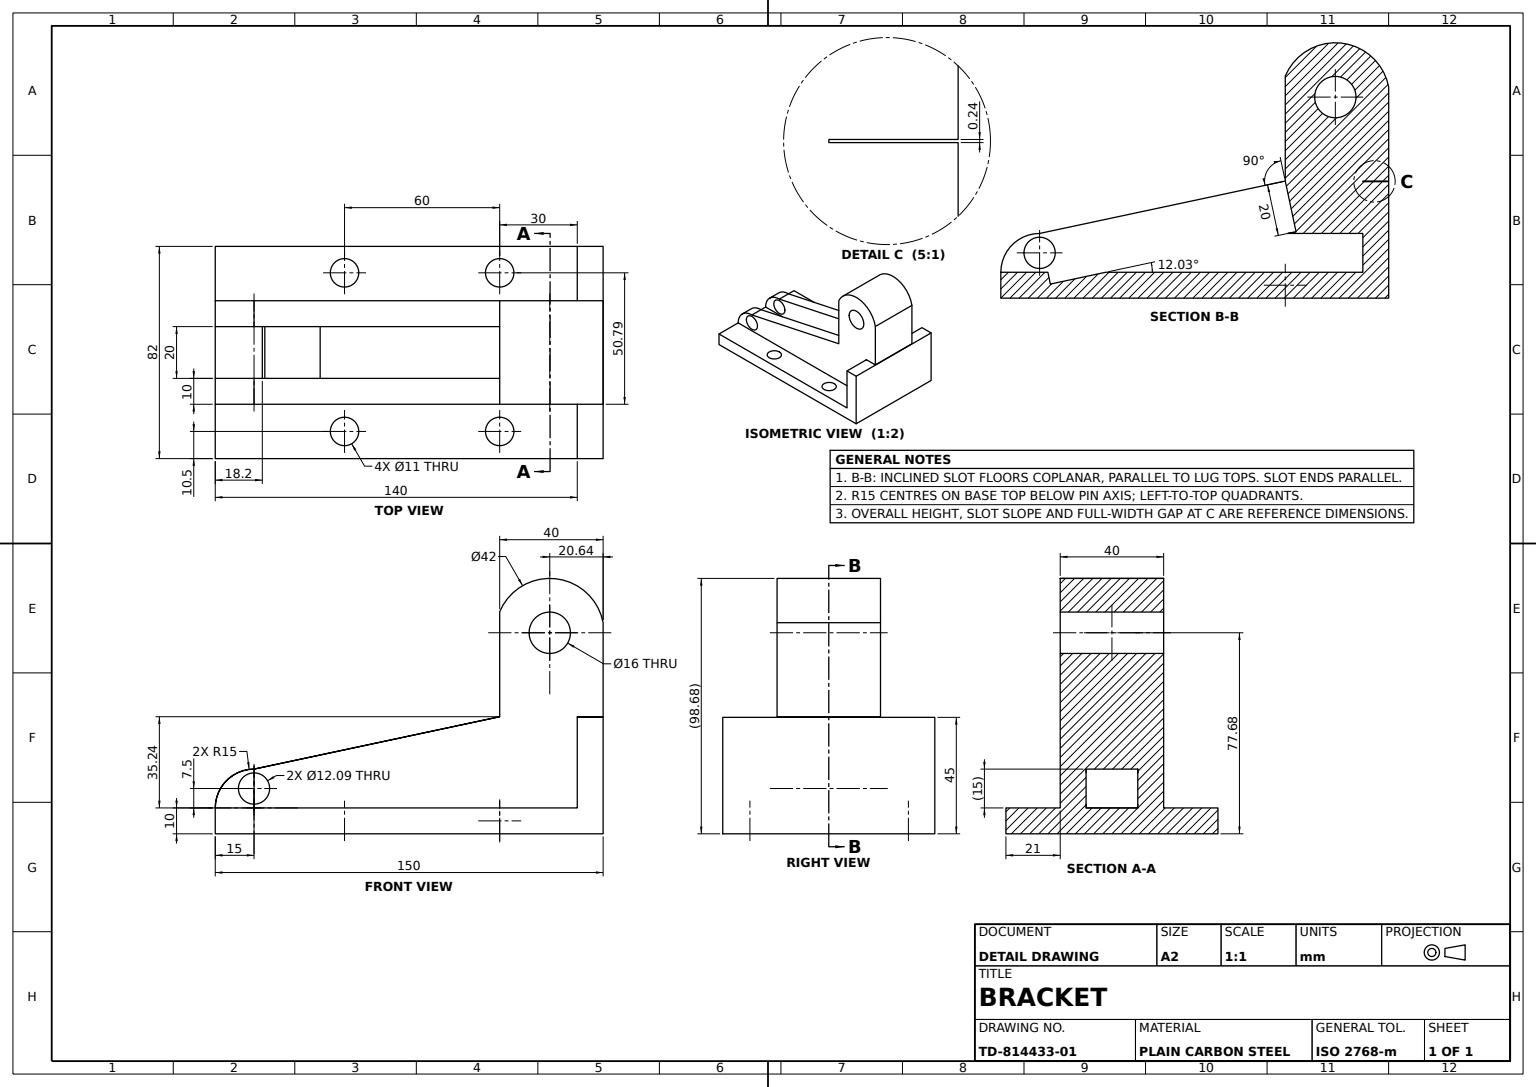
ISO-10303-21;
HEADER;
FILE_DESCRIPTION((''),'2;1');
FILE_NAME('','',(''),(''),'','','');
FILE_SCHEMA(('AUTOMOTIVE_DESIGN'));
ENDSEC;
DATA;
#1=APPLICATION_CONTEXT('');
#2=PRODUCT_CONTEXT('',#1,'mechanical');
#3=PRODUCT('','','',(#2));
#4=PRODUCT_DEFINITION_FORMATION('','',#3);
#5=PRODUCT_DEFINITION_CONTEXT('',#1,'design');
#6=PRODUCT_DEFINITION('','',#4,#5);
#7=PRODUCT_DEFINITION_SHAPE('','',#6);
#8=(LENGTH_UNIT()NAMED_UNIT(*)SI_UNIT(.MILLI.,.METRE.));
#9=(NAMED_UNIT(*)PLANE_ANGLE_UNIT()SI_UNIT($,.RADIAN.));
#10=(NAMED_UNIT(*)SI_UNIT($,.STERADIAN.)SOLID_ANGLE_UNIT());
#11=UNCERTAINTY_MEASURE_WITH_UNIT(LENGTH_MEASURE(1.E-05),#8,'distance_accuracy_value','');
#12=(GEOMETRIC_REPRESENTATION_CONTEXT(3)GLOBAL_UNCERTAINTY_ASSIGNED_CONTEXT((#11))GLOBAL_UNIT_ASSIGNED_CONTEXT((#8,#9,#10))REPRESENTATION_CONTEXT('',''));
#13=CARTESIAN_POINT('',(18.196186,10.,10.));
#14=VERTEX_POINT('',#13);
#15=CARTESIAN_POINT('',(0.,10.,10.));
#16=VERTEX_POINT('',#15);
#17=DIRECTION('',(-1.,0.,0.));
#18=VECTOR('',#17,1000.);
#19=LINE('',#15,#18);
#20=EDGE_CURVE('',#14,#16,#19,.T.);
#21=ORIENTED_EDGE('',*,*,#20,.F.);
#22=CARTESIAN_POINT('',(18.196186,10.,-10.));
#23=VERTEX_POINT('',#22);
#24=CARTESIAN_POINT('',(18.196186,10.,41.));
#25=DIRECTION('',(0.,0.,-1.));
#26=VECTOR('',#25,1000.);
#27=LINE('',#24,#26);
#28=EDGE_CURVE('',#14,#23,#27,.T.);
#29=ORIENTED_EDGE('',*,*,#28,.T.);
#30=CARTESIAN_POINT('',(0.,10.,-10.));
#31=VERTEX_POINT('',#30);
#32=DIRECTION('',(1.,0.,0.));
#33=VECTOR('',#32,1000.);
#34=LINE('',#30,#33);
#35=EDGE_CURVE('',#31,#23,#34,.T.);
#36=ORIENTED_EDGE('',*,*,#35,.F.);
#37=CARTESIAN_POINT('',(0.,10.,41.));
#38=LINE('',#37,#26);
#39=EDGE_CURVE('',#16,#31,#38,.T.);
#40=ORIENTED_EDGE('',*,*,#39,.F.);
#41=EDGE_LOOP('',(#21,#29,#36,#40));
#42=FACE_OUTER_BOUND('',#41,.T.);
#43=DIRECTION('',(0.,-1.,0.));
#44=AXIS2_PLACEMENT_3D('',#37,#43,#25);
#45=PLANE('',#44);
#46=ADVANCED_FACE('',(#42),#45,.F.);
#47=CARTESIAN_POINT('',(110.,45.24251,-10.));
#48=VERTEX_POINT('',#47);
#49=CARTESIAN_POINT('',(15.,25.,-10.));
#50=VERTEX_POINT('',#49);
#51=DIRECTION('',(-0.978043553,-0.208400594,0.));
#52=VECTOR('',#51,1000.);
#53=LINE('',#49,#52);
#54=EDGE_CURVE('',#48,#50,#53,.T.);
#55=ORIENTED_EDGE('',*,*,#54,.F.);
#56=CARTESIAN_POINT('',(110.,45.24251,-20.));
#57=VERTEX_POINT('',#56);
#58=LINE('',#47,#26);
#59=EDGE_CURVE('',#48,#57,#58,.T.);
#60=ORIENTED_EDGE('',*,*,#59,.T.);
#61=CARTESIAN_POINT('',(15.,25.,-20.));
#62=VERTEX_POINT('',#61);
#63=DIRECTION('',(0.978043553,0.208400594,0.));
#64=VECTOR('',#63,1000.);
#65=LINE('',#56,#64);
#66=EDGE_CURVE('',#62,#57,#65,.T.);
#67=ORIENTED_EDGE('',*,*,#66,.F.);
#68=DIRECTION('',(0.,0.,1.));
#69=VECTOR('',#68,1000.);
#70=LINE('',#49,#69);
#71=EDGE_CURVE('',#62,#50,#70,.T.);
#72=ORIENTED_EDGE('',*,*,#71,.T.);
#73=EDGE_LOOP('',(#55,#60,#67,#72));
#74=FACE_OUTER_BOUND('',#73,.T.);
#75=DIRECTION('',(-0.208400594,0.978043553,0.));
#76=AXIS2_PLACEMENT_3D('',#47,#75,#51);
#77=PLANE('',#76);
#78=ADVANCED_FACE('',(#74),#77,.T.);
#79=CARTESIAN_POINT('',(150.,45.,41.));
#80=VERTEX_POINT('',#79);
#81=CARTESIAN_POINT('',(140.,45.,41.));
#82=VERTEX_POINT('',#81);
#83=LINE('',#79,#18);
#84=EDGE_CURVE('',#80,#82,#83,.T.);
#85=ORIENTED_EDGE('',*,*,#84,.T.);
#86=CARTESIAN_POINT('',(140.,10.,41.));
#87=VERTEX_POINT('',#86);
#88=VECTOR('',#43,1000.);
#89=LINE('',#81,#88);
#90=EDGE_CURVE('',#82,#87,#89,.T.);
#91=ORIENTED_EDGE('',*,*,#90,.T.);
#92=VERTEX_POINT('',#37);
#93=LINE('',#37,#18);
#94=EDGE_CURVE('',#87,#92,#93,.T.);
#95=ORIENTED_EDGE('',*,*,#94,.T.);
#96=CARTESIAN_POINT('',(0.,0.,41.));
#97=VERTEX_POINT('',#96);
#98=LINE('',#96,#88);
#99=EDGE_CURVE('',#92,#97,#98,.T.);
#100=ORIENTED_EDGE('',*,*,#99,.T.);
#101=CARTESIAN_POINT('',(150.,0.,41.));
#102=VERTEX_POINT('',#101);
#103=LINE('',#96,#33);
#104=EDGE_CURVE('',#97,#102,#103,.T.);
#105=ORIENTED_EDGE('',*,*,#104,.T.);
#106=DIRECTION('',(0.,1.,0.));
#107=VECTOR('',#106,1000.);
#108=LINE('',#101,#107);
#109=EDGE_CURVE('',#102,#80,#108,.T.);
#110=ORIENTED_EDGE('',*,*,#109,.T.);
#111=EDGE_LOOP('',(#85,#91,#95,#100,#105,#110));
#112=FACE_OUTER_BOUND('',#111,.T.);
#113=AXIS2_PLACEMENT_3D('',#96,#25,#17);
#114=PLANE('',#113);
#115=ADVANCED_FACE('',(#112),#114,.F.);
#116=CARTESIAN_POINT('',(110.,85.812237,-20.));
#117=VERTEX_POINT('',#116);
#118=LINE('',#56,#107);
#119=EDGE_CURVE('',#57,#117,#118,.T.);
#120=ORIENTED_EDGE('',*,*,#119,.F.);
#121=ORIENTED_EDGE('',*,*,#59,.F.);
#122=CARTESIAN_POINT('',(110.,45.24251,10.));
#123=VERTEX_POINT('',#122);
#124=EDGE_CURVE('',#123,#48,#58,.T.);
#125=ORIENTED_EDGE('',*,*,#124,.F.);
#126=CARTESIAN_POINT('',(110.,45.24251,20.));
#127=VERTEX_POINT('',#126);
#128=EDGE_CURVE('',#127,#123,#58,.T.);
#129=ORIENTED_EDGE('',*,*,#128,.F.);
#130=CARTESIAN_POINT('',(110.,85.812237,20.));
#131=VERTEX_POINT('',#130);
#132=LINE('',#126,#107);
#133=EDGE_CURVE('',#127,#131,#132,.T.);
#134=ORIENTED_EDGE('',*,*,#133,.T.);
#135=LINE('',#116,#69);
#136=EDGE_CURVE('',#117,#131,#135,.T.);
#137=ORIENTED_EDGE('',*,*,#136,.F.);
#138=EDGE_LOOP('',(#120,#121,#125,#129,#134,#137));
#139=FACE_OUTER_BOUND('',#138,.T.);
#140=AXIS2_PLACEMENT_3D('',#56,#32,#25);
#141=PLANE('',#140);
#142=ADVANCED_FACE('',(#139),#141,.F.);
#143=CARTESIAN_POINT('',(0.,10.,-20.));
#144=VERTEX_POINT('',#143);
#145=CARTESIAN_POINT('',(0.,10.,-41.));
#146=VERTEX_POINT('',#145);
#147=EDGE_CURVE('',#144,#146,#38,.T.);
#148=ORIENTED_EDGE('',*,*,#147,.F.);
#149=CARTESIAN_POINT('',(140.,10.,-20.));
#150=VERTEX_POINT('',#149);
#151=LINE('',#143,#18);
#152=EDGE_CURVE('',#150,#144,#151,.T.);
#153=ORIENTED_EDGE('',*,*,#152,.F.);
#154=CARTESIAN_POINT('',(140.,10.,-41.));
#155=VERTEX_POINT('',#154);
#156=LINE('',#86,#26);
#157=EDGE_CURVE('',#150,#155,#156,.T.);
#158=ORIENTED_EDGE('',*,*,#157,.T.);
#159=LINE('',#145,#18);
#160=EDGE_CURVE('',#155,#146,#159,.T.);
#161=ORIENTED_EDGE('',*,*,#160,.T.);
#162=EDGE_LOOP('',(#148,#153,#158,#161));
#163=FACE_OUTER_BOUND('',#162,.T.);
#164=CARTESIAN_POINT('',(50.,10.,-25.288669));
#165=VERTEX_POINT('',#164);
#166=CARTESIAN_POINT('',(50.,10.,-36.28851));
#167=VERTEX_POINT('',#166);
#168=CARTESIAN_POINT('',(50.,10.,-30.788589));
#169=AXIS2_PLACEMENT_3D('',#168,#106,#68);
#170=CIRCLE('',#169,5.49992);
#171=EDGE_CURVE('',#165,#167,#170,.T.);
#172=ORIENTED_EDGE('',*,*,#171,.F.);
#173=EDGE_CURVE('',#167,#165,#170,.T.);
#174=ORIENTED_EDGE('',*,*,#173,.F.);
#175=EDGE_LOOP('',(#172,#174));
#176=FACE_BOUND('',#175,.T.);
#177=CARTESIAN_POINT('',(110.,10.,-25.288589));
#178=VERTEX_POINT('',#177);
#179=CARTESIAN_POINT('',(110.,10.,-36.288589));
#180=VERTEX_POINT('',#179);
#181=CARTESIAN_POINT('',(110.,10.,-30.788589));
#182=AXIS2_PLACEMENT_3D('',#181,#106,#68);
#183=CIRCLE('',#182,5.5);
#184=EDGE_CURVE('',#178,#180,#183,.T.);
#185=ORIENTED_EDGE('',*,*,#184,.F.);
#186=EDGE_CURVE('',#180,#178,#183,.T.);
#187=ORIENTED_EDGE('',*,*,#186,.F.);
#188=EDGE_LOOP('',(#185,#187));
#189=FACE_BOUND('',#188,.T.);
#190=ADVANCED_FACE('',(#163,#176,#189),#45,.F.);
#191=CARTESIAN_POINT('',(50.,0.,36.));
#192=VERTEX_POINT('',#191);
#193=CARTESIAN_POINT('',(50.,0.,25.));
#194=VERTEX_POINT('',#193);
#195=CARTESIAN_POINT('',(50.,0.,30.5));
#196=AXIS2_PLACEMENT_3D('',#195,#106,#68);
#197=CIRCLE('',#196,5.5);
#198=EDGE_CURVE('',#192,#194,#197,.T.);
#199=ORIENTED_EDGE('',*,*,#198,.T.);
#200=EDGE_CURVE('',#194,#192,#197,.T.);
#201=ORIENTED_EDGE('',*,*,#200,.T.);
#202=EDGE_LOOP('',(#199,#201));
#203=FACE_BOUND('',#202,.T.);
#204=CARTESIAN_POINT('',(110.,0.,-25.288589));
#205=VERTEX_POINT('',#204);
#206=CARTESIAN_POINT('',(110.,0.,-36.288589));
#207=VERTEX_POINT('',#206);
#208=CARTESIAN_POINT('',(110.,0.,-30.788589));
#209=AXIS2_PLACEMENT_3D('',#208,#106,#68);
#210=CIRCLE('',#209,5.5);
#211=EDGE_CURVE('',#205,#207,#210,.T.);
#212=ORIENTED_EDGE('',*,*,#211,.T.);
#213=EDGE_CURVE('',#207,#205,#210,.T.);
#214=ORIENTED_EDGE('',*,*,#213,.T.);
#215=EDGE_LOOP('',(#212,#214));
#216=FACE_BOUND('',#215,.T.);
#217=CARTESIAN_POINT('',(50.,0.,-25.288669));
#218=VERTEX_POINT('',#217);
#219=CARTESIAN_POINT('',(50.,0.,-36.28851));
#220=VERTEX_POINT('',#219);
#221=CARTESIAN_POINT('',(50.,0.,-30.788589));
#222=AXIS2_PLACEMENT_3D('',#221,#106,#68);
#223=CIRCLE('',#222,5.49992);
#224=EDGE_CURVE('',#218,#220,#223,.T.);
#225=ORIENTED_EDGE('',*,*,#224,.T.);
#226=EDGE_CURVE('',#220,#218,#223,.T.);
#227=ORIENTED_EDGE('',*,*,#226,.T.);
#228=EDGE_LOOP('',(#225,#227));
#229=FACE_BOUND('',#228,.T.);
#230=CARTESIAN_POINT('',(0.,0.,-41.));
#231=VERTEX_POINT('',#230);
#232=LINE('',#96,#26);
#233=EDGE_CURVE('',#97,#231,#232,.T.);
#234=ORIENTED_EDGE('',*,*,#233,.T.);
#235=CARTESIAN_POINT('',(150.,0.,-41.));
#236=VERTEX_POINT('',#235);
#237=LINE('',#230,#33);
#238=EDGE_CURVE('',#231,#236,#237,.T.);
#239=ORIENTED_EDGE('',*,*,#238,.T.);
#240=LINE('',#101,#26);
#241=EDGE_CURVE('',#102,#236,#240,.T.);
#242=ORIENTED_EDGE('',*,*,#241,.F.);
#243=ORIENTED_EDGE('',*,*,#104,.F.);
#244=EDGE_LOOP('',(#234,#239,#242,#243));
#245=FACE_OUTER_BOUND('',#244,.T.);
#246=CARTESIAN_POINT('',(110.,0.,36.));
#247=VERTEX_POINT('',#246);
#248=CARTESIAN_POINT('',(110.,0.,25.));
#249=VERTEX_POINT('',#248);
#250=CARTESIAN_POINT('',(110.,0.,30.5));
#251=AXIS2_PLACEMENT_3D('',#250,#106,#68);
#252=CIRCLE('',#251,5.5);
#253=EDGE_CURVE('',#247,#249,#252,.T.);
#254=ORIENTED_EDGE('',*,*,#253,.T.);
#255=EDGE_CURVE('',#249,#247,#252,.T.);
#256=ORIENTED_EDGE('',*,*,#255,.T.);
#257=EDGE_LOOP('',(#254,#256));
#258=FACE_BOUND('',#257,.T.);
#259=AXIS2_PLACEMENT_3D('',#96,#106,#68);
#260=PLANE('',#259);
#261=ADVANCED_FACE('',(#203,#216,#229,#245,#258),#260,.F.);
#262=CARTESIAN_POINT('',(50.,10.,25.));
#263=VERTEX_POINT('',#262);
#264=CARTESIAN_POINT('',(50.,-70.,25.));
#265=LINE('',#264,#107);
#266=EDGE_CURVE('',#194,#263,#265,.T.);
#267=ORIENTED_EDGE('',*,*,#266,.T.);
#268=CARTESIAN_POINT('',(50.,10.,36.));
#269=VERTEX_POINT('',#268);
#270=CARTESIAN_POINT('',(50.,10.,30.5));
#271=AXIS2_PLACEMENT_3D('',#270,#106,#68);
#272=CIRCLE('',#271,5.5);
#273=EDGE_CURVE('',#263,#269,#272,.T.);
#274=ORIENTED_EDGE('',*,*,#273,.T.);
#275=CARTESIAN_POINT('',(50.,-70.,36.));
#276=LINE('',#275,#107);
#277=EDGE_CURVE('',#192,#269,#276,.T.);
#278=ORIENTED_EDGE('',*,*,#277,.F.);
#279=ORIENTED_EDGE('',*,*,#200,.F.);
#280=EDGE_LOOP('',(#267,#274,#278,#279));
#281=FACE_OUTER_BOUND('',#280,.T.);
#282=CARTESIAN_POINT('',(50.,-70.,30.5));
#283=AXIS2_PLACEMENT_3D('',#282,#106,#68);
#284=CYLINDRICAL_SURFACE('',#283,5.5);
#285=ADVANCED_FACE('',(#281),#284,.F.);
#286=CARTESIAN_POINT('',(150.,45.24251,-20.));
#287=VERTEX_POINT('',#286);
#288=CARTESIAN_POINT('',(150.,45.24251,20.));
#289=VERTEX_POINT('',#288);
#290=LINE('',#286,#69);
#291=EDGE_CURVE('',#287,#289,#290,.T.);
#292=ORIENTED_EDGE('',*,*,#291,.F.);
#293=CARTESIAN_POINT('',(150.,81.572935,-20.));
#294=VERTEX_POINT('',#293);
#295=CARTESIAN_POINT('',(150.,90.24251,-20.));
#296=LINE('',#295,#88);
#297=EDGE_CURVE('',#294,#287,#296,.T.);
#298=ORIENTED_EDGE('',*,*,#297,.F.);
#299=CARTESIAN_POINT('',(150.,81.572935,20.));
#300=VERTEX_POINT('',#299);
#301=LINE('',#293,#69);
#302=EDGE_CURVE('',#294,#300,#301,.T.);
#303=ORIENTED_EDGE('',*,*,#302,.T.);
#304=CARTESIAN_POINT('',(150.,90.24251,20.));
#305=LINE('',#304,#88);
#306=EDGE_CURVE('',#300,#289,#305,.T.);
#307=ORIENTED_EDGE('',*,*,#306,.T.);
#308=EDGE_LOOP('',(#292,#298,#303,#307));
#309=FACE_OUTER_BOUND('',#308,.T.);
#310=AXIS2_PLACEMENT_3D('',#295,#17,#68);
#311=PLANE('',#310);
#312=ADVANCED_FACE('',(#309),#311,.F.);
#313=CARTESIAN_POINT('',(137.363208,77.684128,-20.));
#314=VERTEX_POINT('',#313);
#315=CARTESIAN_POINT('',(137.363208,77.684128,20.));
#316=VERTEX_POINT('',#315);
#317=LINE('',#313,#69);
#318=EDGE_CURVE('',#314,#316,#317,.T.);
#319=ORIENTED_EDGE('',*,*,#318,.F.);
#320=CARTESIAN_POINT('',(121.363208,77.684128,-20.));
#321=VERTEX_POINT('',#320);
#322=CARTESIAN_POINT('',(129.363208,77.684128,-20.));
#323=AXIS2_PLACEMENT_3D('',#322,#68,#32);
#324=CIRCLE('',#323,8.);
#325=EDGE_CURVE('',#321,#314,#324,.T.);
#326=ORIENTED_EDGE('',*,*,#325,.F.);
#327=CARTESIAN_POINT('',(121.363208,77.684128,20.));
#328=VERTEX_POINT('',#327);
#329=LINE('',#320,#69);
#330=EDGE_CURVE('',#321,#328,#329,.T.);
#331=ORIENTED_EDGE('',*,*,#330,.T.);
#332=CARTESIAN_POINT('',(129.363208,77.684128,20.));
#333=AXIS2_PLACEMENT_3D('',#332,#68,#32);
#334=CIRCLE('',#333,8.);
#335=EDGE_CURVE('',#328,#316,#334,.T.);
#336=ORIENTED_EDGE('',*,*,#335,.T.);
#337=EDGE_LOOP('',(#319,#326,#331,#336));
#338=FACE_OUTER_BOUND('',#337,.T.);
#339=CYLINDRICAL_SURFACE('',#323,8.);
#340=ADVANCED_FACE('',(#338),#339,.F.);
#341=ORIENTED_EDGE('',*,*,#152,.T.);
#342=CARTESIAN_POINT('',(15.,10.,-20.));
#343=AXIS2_PLACEMENT_3D('',#342,#25,#32);
#344=CIRCLE('',#343,15.);
#345=EDGE_CURVE('',#144,#62,#344,.T.);
#346=ORIENTED_EDGE('',*,*,#345,.T.);
#347=ORIENTED_EDGE('',*,*,#66,.T.);
#348=ORIENTED_EDGE('',*,*,#119,.T.);
#349=CIRCLE('',#323,21.);
#350=EDGE_CURVE('',#294,#117,#349,.T.);
#351=ORIENTED_EDGE('',*,*,#350,.F.);
#352=ORIENTED_EDGE('',*,*,#297,.T.);
#353=CARTESIAN_POINT('',(140.,45.24251,-20.));
#354=VERTEX_POINT('',#353);
#355=LINE('',#56,#18);
#356=EDGE_CURVE('',#287,#354,#355,.T.);
#357=ORIENTED_EDGE('',*,*,#356,.T.);
#358=CARTESIAN_POINT('',(140.,45.,-20.));
#359=VERTEX_POINT('',#358);
#360=CARTESIAN_POINT('',(140.,25.,-20.));
#361=LINE('',#360,#88);
#362=EDGE_CURVE('',#354,#359,#361,.T.);
#363=ORIENTED_EDGE('',*,*,#362,.T.);
#364=EDGE_CURVE('',#359,#150,#361,.T.);
#365=ORIENTED_EDGE('',*,*,#364,.T.);
#366=EDGE_LOOP('',(#341,#346,#347,#348,#351,#352,#357,#363,#365));
#367=FACE_OUTER_BOUND('',#366,.T.);
#368=CARTESIAN_POINT('',(21.045758,17.5,-20.));
#369=VERTEX_POINT('',#368);
#370=CARTESIAN_POINT('',(8.954242,17.5,-20.));
#371=VERTEX_POINT('',#370);
#372=CARTESIAN_POINT('',(15.,17.5,-20.));
#373=AXIS2_PLACEMENT_3D('',#372,#68,#32);
#374=CIRCLE('',#373,6.045758);
#375=EDGE_CURVE('',#369,#371,#374,.T.);
#376=ORIENTED_EDGE('',*,*,#375,.T.);
#377=EDGE_CURVE('',#371,#369,#374,.T.);
#378=ORIENTED_EDGE('',*,*,#377,.T.);
#379=EDGE_LOOP('',(#376,#378));
#380=FACE_BOUND('',#379,.T.);
#381=ORIENTED_EDGE('',*,*,#325,.T.);
#382=EDGE_CURVE('',#314,#321,#324,.T.);
#383=ORIENTED_EDGE('',*,*,#382,.T.);
#384=EDGE_LOOP('',(#381,#383));
#385=FACE_BOUND('',#384,.T.);
#386=CARTESIAN_POINT('',(0.,25.,-20.));
#387=AXIS2_PLACEMENT_3D('',#386,#68,#32);
#388=PLANE('',#387);
#389=ADVANCED_FACE('',(#367,#380,#385),#388,.F.);
#390=CARTESIAN_POINT('',(140.,25.,10.));
#391=VERTEX_POINT('',#390);
#392=CARTESIAN_POINT('',(110.969016,25.,10.));
#393=VERTEX_POINT('',#392);
#394=CARTESIAN_POINT('',(0.,25.,10.));
#395=LINE('',#394,#18);
#396=EDGE_CURVE('',#391,#393,#395,.T.);
#397=ORIENTED_EDGE('',*,*,#396,.T.);
#398=CARTESIAN_POINT('',(110.969016,25.,-10.));
#399=VERTEX_POINT('',#398);
#400=CARTESIAN_POINT('',(110.969016,25.,20.));
#401=LINE('',#400,#69);
#402=EDGE_CURVE('',#399,#393,#401,.T.);
#403=ORIENTED_EDGE('',*,*,#402,.F.);
#404=CARTESIAN_POINT('',(140.,25.,-10.));
#405=VERTEX_POINT('',#404);
#406=CARTESIAN_POINT('',(0.,25.,-10.));
#407=LINE('',#406,#18);
#408=EDGE_CURVE('',#405,#399,#407,.T.);
#409=ORIENTED_EDGE('',*,*,#408,.F.);
#410=CARTESIAN_POINT('',(140.,25.,20.));
#411=LINE('',#410,#26);
#412=EDGE_CURVE('',#391,#405,#411,.T.);
#413=ORIENTED_EDGE('',*,*,#412,.F.);
#414=EDGE_LOOP('',(#397,#403,#409,#413));
#415=FACE_OUTER_BOUND('',#414,.T.);
#416=CARTESIAN_POINT('',(15.,25.,20.));
#417=AXIS2_PLACEMENT_3D('',#416,#43,#25);
#418=PLANE('',#417);
#419=ADVANCED_FACE('',(#415),#418,.T.);
#420=ORIENTED_EDGE('',*,*,#318,.T.);
#421=EDGE_CURVE('',#316,#328,#334,.T.);
#422=ORIENTED_EDGE('',*,*,#421,.T.);
#423=ORIENTED_EDGE('',*,*,#330,.F.);
#424=ORIENTED_EDGE('',*,*,#382,.F.);
#425=EDGE_LOOP('',(#420,#422,#423,#424));
#426=FACE_OUTER_BOUND('',#425,.T.);
#427=ADVANCED_FACE('',(#426),#339,.F.);
#428=CARTESIAN_POINT('',(50.,-70.,-36.28851));
#429=LINE('',#428,#107);
#430=EDGE_CURVE('',#220,#167,#429,.T.);
#431=ORIENTED_EDGE('',*,*,#430,.F.);
#432=ORIENTED_EDGE('',*,*,#224,.F.);
#433=CARTESIAN_POINT('',(50.,-70.,-25.288669));
#434=LINE('',#433,#107);
#435=EDGE_CURVE('',#218,#165,#434,.T.);
#436=ORIENTED_EDGE('',*,*,#435,.T.);
#437=ORIENTED_EDGE('',*,*,#171,.T.);
#438=EDGE_LOOP('',(#431,#432,#436,#437));
#439=FACE_OUTER_BOUND('',#438,.T.);
#440=CARTESIAN_POINT('',(50.,-70.,-30.788589));
#441=AXIS2_PLACEMENT_3D('',#440,#106,#68);
#442=CYLINDRICAL_SURFACE('',#441,5.49992);
#443=ADVANCED_FACE('',(#439),#442,.F.);
#444=ORIENTED_EDGE('',*,*,#302,.F.);
#445=ORIENTED_EDGE('',*,*,#350,.T.);
#446=ORIENTED_EDGE('',*,*,#136,.T.);
#447=CIRCLE('',#333,21.);
#448=EDGE_CURVE('',#300,#131,#447,.T.);
#449=ORIENTED_EDGE('',*,*,#448,.F.);
#450=EDGE_LOOP('',(#444,#445,#446,#449));
#451=FACE_OUTER_BOUND('',#450,.T.);
#452=CYLINDRICAL_SURFACE('',#323,21.);
#453=ADVANCED_FACE('',(#451),#452,.T.);
#454=CARTESIAN_POINT('',(140.,10.,-10.));
#455=VERTEX_POINT('',#454);
#456=LINE('',#404,#88);
#457=EDGE_CURVE('',#405,#455,#456,.T.);
#458=ORIENTED_EDGE('',*,*,#457,.T.);
#459=CARTESIAN_POINT('',(140.,10.,10.));
#460=VERTEX_POINT('',#459);
#461=EDGE_CURVE('',#460,#455,#156,.T.);
#462=ORIENTED_EDGE('',*,*,#461,.F.);
#463=LINE('',#390,#88);
#464=EDGE_CURVE('',#391,#460,#463,.T.);
#465=ORIENTED_EDGE('',*,*,#464,.F.);
#466=ORIENTED_EDGE('',*,*,#412,.T.);
#467=EDGE_LOOP('',(#458,#462,#465,#466));
#468=FACE_OUTER_BOUND('',#467,.T.);
#469=AXIS2_PLACEMENT_3D('',#81,#32,#106);
#470=PLANE('',#469);
#471=ADVANCED_FACE('',(#468),#470,.F.);
#472=ORIENTED_EDGE('',*,*,#198,.F.);
#473=ORIENTED_EDGE('',*,*,#277,.T.);
#474=EDGE_CURVE('',#269,#263,#272,.T.);
#475=ORIENTED_EDGE('',*,*,#474,.T.);
#476=ORIENTED_EDGE('',*,*,#266,.F.);
#477=EDGE_LOOP('',(#472,#473,#475,#476));
#478=FACE_OUTER_BOUND('',#477,.T.);
#479=ADVANCED_FACE('',(#478),#284,.F.);
#480=CARTESIAN_POINT('',(114.168012,25.681639,-10.));
#481=VERTEX_POINT('',#480);
#482=VECTOR('',#75,1000.);
#483=LINE('',#480,#482);
#484=EDGE_CURVE('',#481,#48,#483,.T.);
#485=ORIENTED_EDGE('',*,*,#484,.F.);
#486=CARTESIAN_POINT('',(114.168012,25.681639,10.));
#487=VERTEX_POINT('',#486);
#488=LINE('',#480,#26);
#489=EDGE_CURVE('',#487,#481,#488,.T.);
#490=ORIENTED_EDGE('',*,*,#489,.F.);
#491=LINE('',#486,#482);
#492=EDGE_CURVE('',#487,#123,#491,.T.);
#493=ORIENTED_EDGE('',*,*,#492,.T.);
#494=ORIENTED_EDGE('',*,*,#124,.T.);
#495=EDGE_LOOP('',(#485,#490,#493,#494));
#496=FACE_OUTER_BOUND('',#495,.T.);
#497=AXIS2_PLACEMENT_3D('',#480,#63,#75);
#498=PLANE('',#497);
#499=ADVANCED_FACE('',(#496),#498,.F.);
#500=CARTESIAN_POINT('',(8.954242,17.5,-10.));
#501=VERTEX_POINT('',#500);
#502=CARTESIAN_POINT('',(21.045758,17.5,-10.));
#503=VERTEX_POINT('',#502);
#504=CARTESIAN_POINT('',(15.,17.5,-10.));
#505=AXIS2_PLACEMENT_3D('',#504,#25,#17);
#506=CIRCLE('',#505,6.045758);
#507=EDGE_CURVE('',#501,#503,#506,.T.);
#508=ORIENTED_EDGE('',*,*,#507,.F.);
#509=CARTESIAN_POINT('',(8.954242,17.5,-60.));
#510=LINE('',#509,#69);
#511=EDGE_CURVE('',#371,#501,#510,.T.);
#512=ORIENTED_EDGE('',*,*,#511,.F.);
#513=ORIENTED_EDGE('',*,*,#375,.F.);
#514=CARTESIAN_POINT('',(21.045758,17.5,-60.));
#515=LINE('',#514,#69);
#516=EDGE_CURVE('',#369,#503,#515,.T.);
#517=ORIENTED_EDGE('',*,*,#516,.T.);
#518=EDGE_LOOP('',(#508,#512,#513,#517));
#519=FACE_OUTER_BOUND('',#518,.T.);
#520=CARTESIAN_POINT('',(15.,17.5,-60.));
#521=AXIS2_PLACEMENT_3D('',#520,#68,#32);
#522=CYLINDRICAL_SURFACE('',#521,6.045758);
#523=ADVANCED_FACE('',(#519),#522,.F.);
#524=CARTESIAN_POINT('',(21.045758,17.5,10.));
#525=VERTEX_POINT('',#524);
#526=CARTESIAN_POINT('',(8.954242,17.5,10.));
#527=VERTEX_POINT('',#526);
#528=CARTESIAN_POINT('',(15.,17.5,10.));
#529=AXIS2_PLACEMENT_3D('',#528,#68,#32);
#530=CIRCLE('',#529,6.045758);
#531=EDGE_CURVE('',#525,#527,#530,.T.);
#532=ORIENTED_EDGE('',*,*,#531,.T.);
#533=EDGE_CURVE('',#527,#525,#530,.T.);
#534=ORIENTED_EDGE('',*,*,#533,.T.);
#535=EDGE_LOOP('',(#532,#534));
#536=FACE_BOUND('',#535,.T.);
#537=CARTESIAN_POINT('',(40.572608,10.,10.));
#538=VERTEX_POINT('',#537);
#539=EDGE_CURVE('',#460,#538,#19,.T.);
#540=ORIENTED_EDGE('',*,*,#539,.T.);
#541=CARTESIAN_POINT('',(19.168012,5.439129,10.));
#542=VERTEX_POINT('',#541);
#543=LINE('',#486,#64);
#544=EDGE_CURVE('',#542,#538,#543,.T.);
#545=ORIENTED_EDGE('',*,*,#544,.F.);
#546=LINE('',#541,#482);
#547=EDGE_CURVE('',#542,#14,#546,.T.);
#548=ORIENTED_EDGE('',*,*,#547,.T.);
#549=ORIENTED_EDGE('',*,*,#20,.T.);
#550=CARTESIAN_POINT('',(15.,25.,10.));
#551=VERTEX_POINT('',#550);
#552=CARTESIAN_POINT('',(15.,10.,10.));
#553=AXIS2_PLACEMENT_3D('',#552,#25,#32);
#554=CIRCLE('',#553,15.);
#555=EDGE_CURVE('',#16,#551,#554,.T.);
#556=ORIENTED_EDGE('',*,*,#555,.T.);
#557=LINE('',#122,#64);
#558=EDGE_CURVE('',#551,#123,#557,.T.);
#559=ORIENTED_EDGE('',*,*,#558,.T.);
#560=ORIENTED_EDGE('',*,*,#492,.F.);
#561=EDGE_CURVE('',#393,#487,#543,.T.);
#562=ORIENTED_EDGE('',*,*,#561,.F.);
#563=ORIENTED_EDGE('',*,*,#396,.F.);
#564=ORIENTED_EDGE('',*,*,#464,.T.);
#565=EDGE_LOOP('',(#540,#545,#548,#549,#556,#559,#560,#562,#563,#564));
#566=FACE_OUTER_BOUND('',#565,.T.);
#567=AXIS2_PLACEMENT_3D('',#394,#68,#32);
#568=PLANE('',#567);
#569=ADVANCED_FACE('',(#536,#566),#568,.F.);
#570=ORIENTED_EDGE('',*,*,#547,.F.);
#571=CARTESIAN_POINT('',(19.168012,5.439129,-10.));
#572=VERTEX_POINT('',#571);
#573=LINE('',#541,#69);
#574=EDGE_CURVE('',#572,#542,#573,.T.);
#575=ORIENTED_EDGE('',*,*,#574,.F.);
#576=LINE('',#571,#482);
#577=EDGE_CURVE('',#572,#23,#576,.T.);
#578=ORIENTED_EDGE('',*,*,#577,.T.);
#579=ORIENTED_EDGE('',*,*,#28,.F.);
#580=EDGE_LOOP('',(#570,#575,#578,#579));
#581=FACE_OUTER_BOUND('',#580,.T.);
#582=DIRECTION('',(0.208400594,-0.978043553,0.));
#583=AXIS2_PLACEMENT_3D('',#541,#51,#582);
#584=PLANE('',#583);
#585=ADVANCED_FACE('',(#581),#584,.F.);
#586=EDGE_CURVE('',#503,#501,#506,.T.);
#587=ORIENTED_EDGE('',*,*,#586,.F.);
#588=ORIENTED_EDGE('',*,*,#516,.F.);
#589=ORIENTED_EDGE('',*,*,#377,.F.);
#590=ORIENTED_EDGE('',*,*,#511,.T.);
#591=EDGE_LOOP('',(#587,#588,#589,#590));
#592=FACE_OUTER_BOUND('',#591,.T.);
#593=ADVANCED_FACE('',(#592),#522,.F.);
#594=CARTESIAN_POINT('',(15.,10.,-10.));
#595=AXIS2_PLACEMENT_3D('',#594,#68,#17);
#596=CIRCLE('',#595,15.);
#597=EDGE_CURVE('',#50,#31,#596,.T.);
#598=ORIENTED_EDGE('',*,*,#597,.F.);
#599=ORIENTED_EDGE('',*,*,#71,.F.);
#600=ORIENTED_EDGE('',*,*,#345,.F.);
#601=LINE('',#143,#26);
#602=EDGE_CURVE('',#31,#144,#601,.T.);
#603=ORIENTED_EDGE('',*,*,#602,.F.);
#604=EDGE_LOOP('',(#598,#599,#600,#603));
#605=FACE_OUTER_BOUND('',#604,.T.);
#606=CARTESIAN_POINT('',(15.,10.,0.));
#607=AXIS2_PLACEMENT_3D('',#606,#25,#17);
#608=CYLINDRICAL_SURFACE('',#607,15.);
#609=ADVANCED_FACE('',(#605),#608,.T.);
#610=ORIENTED_EDGE('',*,*,#586,.T.);
#611=ORIENTED_EDGE('',*,*,#507,.T.);
#612=EDGE_LOOP('',(#610,#611));
#613=FACE_BOUND('',#612,.T.);
#614=LINE('',#571,#52);
#615=EDGE_CURVE('',#481,#399,#614,.T.);
#616=ORIENTED_EDGE('',*,*,#615,.F.);
#617=ORIENTED_EDGE('',*,*,#484,.T.);
#618=ORIENTED_EDGE('',*,*,#54,.T.);
#619=ORIENTED_EDGE('',*,*,#597,.T.);
#620=ORIENTED_EDGE('',*,*,#35,.T.);
#621=ORIENTED_EDGE('',*,*,#577,.F.);
#622=CARTESIAN_POINT('',(40.572608,10.,-10.));
#623=VERTEX_POINT('',#622);
#624=EDGE_CURVE('',#623,#572,#614,.T.);
#625=ORIENTED_EDGE('',*,*,#624,.F.);
#626=EDGE_CURVE('',#623,#455,#34,.T.);
#627=ORIENTED_EDGE('',*,*,#626,.T.);
#628=ORIENTED_EDGE('',*,*,#457,.F.);
#629=ORIENTED_EDGE('',*,*,#408,.T.);
#630=EDGE_LOOP('',(#616,#617,#618,#619,#620,#621,#625,#627,#628,#629));
#631=FACE_OUTER_BOUND('',#630,.T.);
#632=AXIS2_PLACEMENT_3D('',#406,#25,#17);
#633=PLANE('',#632);
#634=ADVANCED_FACE('',(#613,#631),#633,.F.);
#635=CARTESIAN_POINT('',(150.,45.,-41.));
#636=VERTEX_POINT('',#635);
#637=LINE('',#79,#26);
#638=EDGE_CURVE('',#80,#636,#637,.T.);
#639=ORIENTED_EDGE('',*,*,#638,.T.);
#640=CARTESIAN_POINT('',(140.,45.,-41.));
#641=VERTEX_POINT('',#640);
#642=LINE('',#635,#18);
#643=EDGE_CURVE('',#636,#641,#642,.T.);
#644=ORIENTED_EDGE('',*,*,#643,.T.);
#645=LINE('',#81,#26);
#646=EDGE_CURVE('',#359,#641,#645,.T.);
#647=ORIENTED_EDGE('',*,*,#646,.F.);
#648=CARTESIAN_POINT('',(140.,45.,20.));
#649=VERTEX_POINT('',#648);
#650=LINE('',#81,#69);
#651=EDGE_CURVE('',#359,#649,#650,.T.);
#652=ORIENTED_EDGE('',*,*,#651,.T.);
#653=EDGE_CURVE('',#82,#649,#645,.T.);
#654=ORIENTED_EDGE('',*,*,#653,.F.);
#655=ORIENTED_EDGE('',*,*,#84,.F.);
#656=EDGE_LOOP('',(#639,#644,#647,#652,#654,#655));
#657=FACE_OUTER_BOUND('',#656,.T.);
#658=AXIS2_PLACEMENT_3D('',#79,#43,#25);
#659=PLANE('',#658);
#660=ADVANCED_FACE('',(#657),#659,.F.);
#661=CARTESIAN_POINT('',(0.,10.,20.));
#662=VERTEX_POINT('',#661);
#663=LINE('',#15,#26);
#664=EDGE_CURVE('',#662,#16,#663,.T.);
#665=ORIENTED_EDGE('',*,*,#664,.F.);
#666=VERTEX_POINT('',#416);
#667=CARTESIAN_POINT('',(15.,10.,20.));
#668=AXIS2_PLACEMENT_3D('',#667,#68,#17);
#669=CIRCLE('',#668,15.);
#670=EDGE_CURVE('',#666,#662,#669,.T.);
#671=ORIENTED_EDGE('',*,*,#670,.F.);
#672=LINE('',#416,#69);
#673=EDGE_CURVE('',#551,#666,#672,.T.);
#674=ORIENTED_EDGE('',*,*,#673,.F.);
#675=ORIENTED_EDGE('',*,*,#555,.F.);
#676=EDGE_LOOP('',(#665,#671,#674,#675));
#677=FACE_OUTER_BOUND('',#676,.T.);
#678=ADVANCED_FACE('',(#677),#608,.T.);
#679=ORIENTED_EDGE('',*,*,#213,.F.);
#680=CARTESIAN_POINT('',(110.,-70.,-36.288589));
#681=LINE('',#680,#107);
#682=EDGE_CURVE('',#207,#180,#681,.T.);
#683=ORIENTED_EDGE('',*,*,#682,.T.);
#684=ORIENTED_EDGE('',*,*,#186,.T.);
#685=CARTESIAN_POINT('',(110.,-70.,-25.288589));
#686=LINE('',#685,#107);
#687=EDGE_CURVE('',#205,#178,#686,.T.);
#688=ORIENTED_EDGE('',*,*,#687,.F.);
#689=EDGE_LOOP('',(#679,#683,#684,#688));
#690=FACE_OUTER_BOUND('',#689,.T.);
#691=CARTESIAN_POINT('',(110.,-70.,-30.788589));
#692=AXIS2_PLACEMENT_3D('',#691,#106,#68);
#693=CYLINDRICAL_SURFACE('',#692,5.5);
#694=ADVANCED_FACE('',(#690),#693,.F.);
#695=ORIENTED_EDGE('',*,*,#626,.F.);
#696=CARTESIAN_POINT('',(40.572608,10.,41.));
#697=LINE('',#696,#69);
#698=EDGE_CURVE('',#623,#538,#697,.T.);
#699=ORIENTED_EDGE('',*,*,#698,.T.);
#700=ORIENTED_EDGE('',*,*,#539,.F.);
#701=ORIENTED_EDGE('',*,*,#461,.T.);
#702=EDGE_LOOP('',(#695,#699,#700,#701));
#703=FACE_OUTER_BOUND('',#702,.T.);
#704=ADVANCED_FACE('',(#703),#45,.F.);
#705=ORIENTED_EDGE('',*,*,#184,.T.);
#706=ORIENTED_EDGE('',*,*,#682,.F.);
#707=ORIENTED_EDGE('',*,*,#211,.F.);
#708=ORIENTED_EDGE('',*,*,#687,.T.);
#709=EDGE_LOOP('',(#705,#706,#707,#708));
#710=FACE_OUTER_BOUND('',#709,.T.);
#711=ADVANCED_FACE('',(#710),#693,.F.);
#712=LINE('',#126,#64);
#713=EDGE_CURVE('',#666,#127,#712,.T.);
#714=ORIENTED_EDGE('',*,*,#713,.T.);
#715=ORIENTED_EDGE('',*,*,#128,.T.);
#716=ORIENTED_EDGE('',*,*,#558,.F.);
#717=ORIENTED_EDGE('',*,*,#673,.T.);
#718=EDGE_LOOP('',(#714,#715,#716,#717));
#719=FACE_OUTER_BOUND('',#718,.T.);
#720=ADVANCED_FACE('',(#719),#77,.T.);
#721=ORIENTED_EDGE('',*,*,#544,.T.);
#722=ORIENTED_EDGE('',*,*,#698,.F.);
#723=ORIENTED_EDGE('',*,*,#624,.T.);
#724=ORIENTED_EDGE('',*,*,#574,.T.);
#725=EDGE_LOOP('',(#721,#722,#723,#724));
#726=FACE_OUTER_BOUND('',#725,.T.);
#727=CARTESIAN_POINT('',(-0.276147,1.295986,0.));
#728=AXIS2_PLACEMENT_3D('',#727,#582,#63);
#729=PLANE('',#728);
#730=ADVANCED_FACE('',(#726),#729,.F.);
#731=ORIENTED_EDGE('',*,*,#651,.F.);
#732=ORIENTED_EDGE('',*,*,#362,.F.);
#733=CARTESIAN_POINT('',(140.,45.24251,20.));
#734=VERTEX_POINT('',#733);
#735=CARTESIAN_POINT('',(140.,45.24251,-10.));
#736=LINE('',#735,#26);
#737=EDGE_CURVE('',#734,#354,#736,.T.);
#738=ORIENTED_EDGE('',*,*,#737,.F.);
#739=LINE('',#410,#88);
#740=EDGE_CURVE('',#734,#649,#739,.T.);
#741=ORIENTED_EDGE('',*,*,#740,.T.);
#742=EDGE_LOOP('',(#731,#732,#738,#741));
#743=FACE_OUTER_BOUND('',#742,.T.);
#744=AXIS2_PLACEMENT_3D('',#404,#32,#25);
#745=PLANE('',#744);
#746=ADVANCED_FACE('',(#743),#745,.T.);
#747=ORIENTED_EDGE('',*,*,#615,.T.);
#748=ORIENTED_EDGE('',*,*,#402,.T.);
#749=ORIENTED_EDGE('',*,*,#561,.T.);
#750=ORIENTED_EDGE('',*,*,#489,.T.);
#751=EDGE_LOOP('',(#747,#748,#749,#750));
#752=FACE_OUTER_BOUND('',#751,.T.);
#753=ADVANCED_FACE('',(#752),#729,.F.);
#754=ORIENTED_EDGE('',*,*,#646,.T.);
#755=LINE('',#640,#88);
#756=EDGE_CURVE('',#641,#155,#755,.T.);
#757=ORIENTED_EDGE('',*,*,#756,.T.);
#758=ORIENTED_EDGE('',*,*,#157,.F.);
#759=ORIENTED_EDGE('',*,*,#364,.F.);
#760=EDGE_LOOP('',(#754,#757,#758,#759));
#761=FACE_OUTER_BOUND('',#760,.T.);
#762=ADVANCED_FACE('',(#761),#470,.F.);
#763=ORIENTED_EDGE('',*,*,#173,.T.);
#764=ORIENTED_EDGE('',*,*,#435,.F.);
#765=ORIENTED_EDGE('',*,*,#226,.F.);
#766=ORIENTED_EDGE('',*,*,#430,.T.);
#767=EDGE_LOOP('',(#763,#764,#765,#766));
#768=FACE_OUTER_BOUND('',#767,.T.);
#769=ADVANCED_FACE('',(#768),#442,.F.);
#770=ORIENTED_EDGE('',*,*,#653,.T.);
#771=CARTESIAN_POINT('',(140.,10.,20.));
#772=VERTEX_POINT('',#771);
#773=EDGE_CURVE('',#649,#772,#739,.T.);
#774=ORIENTED_EDGE('',*,*,#773,.T.);
#775=EDGE_CURVE('',#87,#772,#156,.T.);
#776=ORIENTED_EDGE('',*,*,#775,.F.);
#777=ORIENTED_EDGE('',*,*,#90,.F.);
#778=EDGE_LOOP('',(#770,#774,#776,#777));
#779=FACE_OUTER_BOUND('',#778,.T.);
#780=ADVANCED_FACE('',(#779),#470,.F.);
#781=ORIENTED_EDGE('',*,*,#474,.F.);
#782=ORIENTED_EDGE('',*,*,#273,.F.);
#783=EDGE_LOOP('',(#781,#782));
#784=FACE_BOUND('',#783,.T.);
#785=LINE('',#661,#33);
#786=EDGE_CURVE('',#662,#772,#785,.T.);
#787=ORIENTED_EDGE('',*,*,#786,.F.);
#788=EDGE_CURVE('',#92,#662,#38,.T.);
#789=ORIENTED_EDGE('',*,*,#788,.F.);
#790=ORIENTED_EDGE('',*,*,#94,.F.);
#791=ORIENTED_EDGE('',*,*,#775,.T.);
#792=EDGE_LOOP('',(#787,#789,#790,#791));
#793=FACE_OUTER_BOUND('',#792,.T.);
#794=CARTESIAN_POINT('',(110.,10.,25.));
#795=VERTEX_POINT('',#794);
#796=CARTESIAN_POINT('',(110.,10.,36.));
#797=VERTEX_POINT('',#796);
#798=CARTESIAN_POINT('',(110.,10.,30.5));
#799=AXIS2_PLACEMENT_3D('',#798,#106,#68);
#800=CIRCLE('',#799,5.5);
#801=EDGE_CURVE('',#795,#797,#800,.T.);
#802=ORIENTED_EDGE('',*,*,#801,.F.);
#803=EDGE_CURVE('',#797,#795,#800,.T.);
#804=ORIENTED_EDGE('',*,*,#803,.F.);
#805=EDGE_LOOP('',(#802,#804));
#806=FACE_BOUND('',#805,.T.);
#807=ADVANCED_FACE('',(#784,#793,#806),#45,.F.);
#808=ORIENTED_EDGE('',*,*,#253,.F.);
#809=CARTESIAN_POINT('',(110.,-70.,36.));
#810=LINE('',#809,#107);
#811=EDGE_CURVE('',#247,#797,#810,.T.);
#812=ORIENTED_EDGE('',*,*,#811,.T.);
#813=ORIENTED_EDGE('',*,*,#803,.T.);
#814=CARTESIAN_POINT('',(110.,-70.,25.));
#815=LINE('',#814,#107);
#816=EDGE_CURVE('',#249,#795,#815,.T.);
#817=ORIENTED_EDGE('',*,*,#816,.F.);
#818=EDGE_LOOP('',(#808,#812,#813,#817));
#819=FACE_OUTER_BOUND('',#818,.T.);
#820=CARTESIAN_POINT('',(110.,-70.,30.5));
#821=AXIS2_PLACEMENT_3D('',#820,#106,#68);
#822=CYLINDRICAL_SURFACE('',#821,5.5);
#823=ADVANCED_FACE('',(#819),#822,.F.);
#824=CARTESIAN_POINT('',(8.954242,17.5,20.));
#825=VERTEX_POINT('',#824);
#826=EDGE_CURVE('',#527,#825,#510,.T.);
#827=ORIENTED_EDGE('',*,*,#826,.F.);
#828=ORIENTED_EDGE('',*,*,#531,.F.);
#829=CARTESIAN_POINT('',(21.045758,17.5,20.));
#830=VERTEX_POINT('',#829);
#831=EDGE_CURVE('',#525,#830,#515,.T.);
#832=ORIENTED_EDGE('',*,*,#831,.T.);
#833=CARTESIAN_POINT('',(15.,17.5,20.));
#834=AXIS2_PLACEMENT_3D('',#833,#68,#32);
#835=CIRCLE('',#834,6.045758);
#836=EDGE_CURVE('',#830,#825,#835,.T.);
#837=ORIENTED_EDGE('',*,*,#836,.T.);
#838=EDGE_LOOP('',(#827,#828,#832,#837));
#839=FACE_OUTER_BOUND('',#838,.T.);
#840=ADVANCED_FACE('',(#839),#522,.F.);
#841=ORIENTED_EDGE('',*,*,#291,.T.);
#842=LINE('',#126,#18);
#843=EDGE_CURVE('',#289,#734,#842,.T.);
#844=ORIENTED_EDGE('',*,*,#843,.T.);
#845=ORIENTED_EDGE('',*,*,#737,.T.);
#846=ORIENTED_EDGE('',*,*,#356,.F.);
#847=EDGE_LOOP('',(#841,#844,#845,#846));
#848=FACE_OUTER_BOUND('',#847,.T.);
#849=AXIS2_PLACEMENT_3D('',#56,#106,#68);
#850=PLANE('',#849);
#851=ADVANCED_FACE('',(#848),#850,.F.);
#852=LINE('',#235,#107);
#853=EDGE_CURVE('',#236,#636,#852,.T.);
#854=ORIENTED_EDGE('',*,*,#853,.T.);
#855=ORIENTED_EDGE('',*,*,#638,.F.);
#856=ORIENTED_EDGE('',*,*,#109,.F.);
#857=ORIENTED_EDGE('',*,*,#241,.T.);
#858=EDGE_LOOP('',(#854,#855,#856,#857));
#859=FACE_OUTER_BOUND('',#858,.T.);
#860=AXIS2_PLACEMENT_3D('',#101,#17,#68);
#861=PLANE('',#860);
#862=ADVANCED_FACE('',(#859),#861,.F.);
#863=ORIENTED_EDGE('',*,*,#801,.T.);
#864=ORIENTED_EDGE('',*,*,#811,.F.);
#865=ORIENTED_EDGE('',*,*,#255,.F.);
#866=ORIENTED_EDGE('',*,*,#816,.T.);
#867=EDGE_LOOP('',(#863,#864,#865,#866));
#868=FACE_OUTER_BOUND('',#867,.T.);
#869=ADVANCED_FACE('',(#868),#822,.F.);
#870=EDGE_CURVE('',#825,#830,#835,.T.);
#871=ORIENTED_EDGE('',*,*,#870,.F.);
#872=ORIENTED_EDGE('',*,*,#836,.F.);
#873=EDGE_LOOP('',(#871,#872));
#874=FACE_BOUND('',#873,.T.);
#875=ORIENTED_EDGE('',*,*,#335,.F.);
#876=ORIENTED_EDGE('',*,*,#421,.F.);
#877=EDGE_LOOP('',(#875,#876));
#878=FACE_BOUND('',#877,.T.);
#879=ORIENTED_EDGE('',*,*,#786,.T.);
#880=ORIENTED_EDGE('',*,*,#773,.F.);
#881=ORIENTED_EDGE('',*,*,#740,.F.);
#882=ORIENTED_EDGE('',*,*,#843,.F.);
#883=ORIENTED_EDGE('',*,*,#306,.F.);
#884=ORIENTED_EDGE('',*,*,#448,.T.);
#885=ORIENTED_EDGE('',*,*,#133,.F.);
#886=ORIENTED_EDGE('',*,*,#713,.F.);
#887=ORIENTED_EDGE('',*,*,#670,.T.);
#888=EDGE_LOOP('',(#879,#880,#881,#882,#883,#884,#885,#886,#887));
#889=FACE_OUTER_BOUND('',#888,.T.);
#890=CARTESIAN_POINT('',(0.,25.,20.));
#891=AXIS2_PLACEMENT_3D('',#890,#25,#17);
#892=PLANE('',#891);
#893=ADVANCED_FACE('',(#874,#878,#889),#892,.F.);
#894=LINE('',#230,#88);
#895=EDGE_CURVE('',#146,#231,#894,.T.);
#896=ORIENTED_EDGE('',*,*,#895,.F.);
#897=ORIENTED_EDGE('',*,*,#160,.F.);
#898=ORIENTED_EDGE('',*,*,#756,.F.);
#899=ORIENTED_EDGE('',*,*,#643,.F.);
#900=ORIENTED_EDGE('',*,*,#853,.F.);
#901=ORIENTED_EDGE('',*,*,#238,.F.);
#902=EDGE_LOOP('',(#896,#897,#898,#899,#900,#901));
#903=FACE_OUTER_BOUND('',#902,.T.);
#904=AXIS2_PLACEMENT_3D('',#230,#25,#17);
#905=PLANE('',#904);
#906=ADVANCED_FACE('',(#903),#905,.T.);
#907=ORIENTED_EDGE('',*,*,#99,.F.);
#908=ORIENTED_EDGE('',*,*,#788,.T.);
#909=ORIENTED_EDGE('',*,*,#664,.T.);
#910=ORIENTED_EDGE('',*,*,#39,.T.);
#911=ORIENTED_EDGE('',*,*,#602,.T.);
#912=ORIENTED_EDGE('',*,*,#147,.T.);
#913=ORIENTED_EDGE('',*,*,#895,.T.);
#914=ORIENTED_EDGE('',*,*,#233,.F.);
#915=EDGE_LOOP('',(#907,#908,#909,#910,#911,#912,#913,#914));
#916=FACE_OUTER_BOUND('',#915,.T.);
#917=AXIS2_PLACEMENT_3D('',#96,#32,#25);
#918=PLANE('',#917);
#919=ADVANCED_FACE('',(#916),#918,.F.);
#920=ORIENTED_EDGE('',*,*,#533,.F.);
#921=ORIENTED_EDGE('',*,*,#826,.T.);
#922=ORIENTED_EDGE('',*,*,#870,.T.);
#923=ORIENTED_EDGE('',*,*,#831,.F.);
#924=EDGE_LOOP('',(#920,#921,#922,#923));
#925=FACE_OUTER_BOUND('',#924,.T.);
#926=ADVANCED_FACE('',(#925),#522,.F.);
#927=CLOSED_SHELL('',(#46,#78,#115,#142,#190,#261,#285,#312,#340,#389,#419,#427,#443,#453,#471,#479,#499,#523,#569,#585,#593,#609,#634,#660,#678,#694,#704,#711,#720,#730,#746,#753,#762,#769,#780,#807,#823,#840,#851,#862,#869,#893,#906,#919,#926));
#928=MANIFOLD_SOLID_BREP('',#927);
#929=ADVANCED_BREP_SHAPE_REPRESENTATION('',(#928),#12);
#930=SHAPE_DEFINITION_REPRESENTATION(#7,#929);
ENDSEC;
END-ISO-10303-21;
